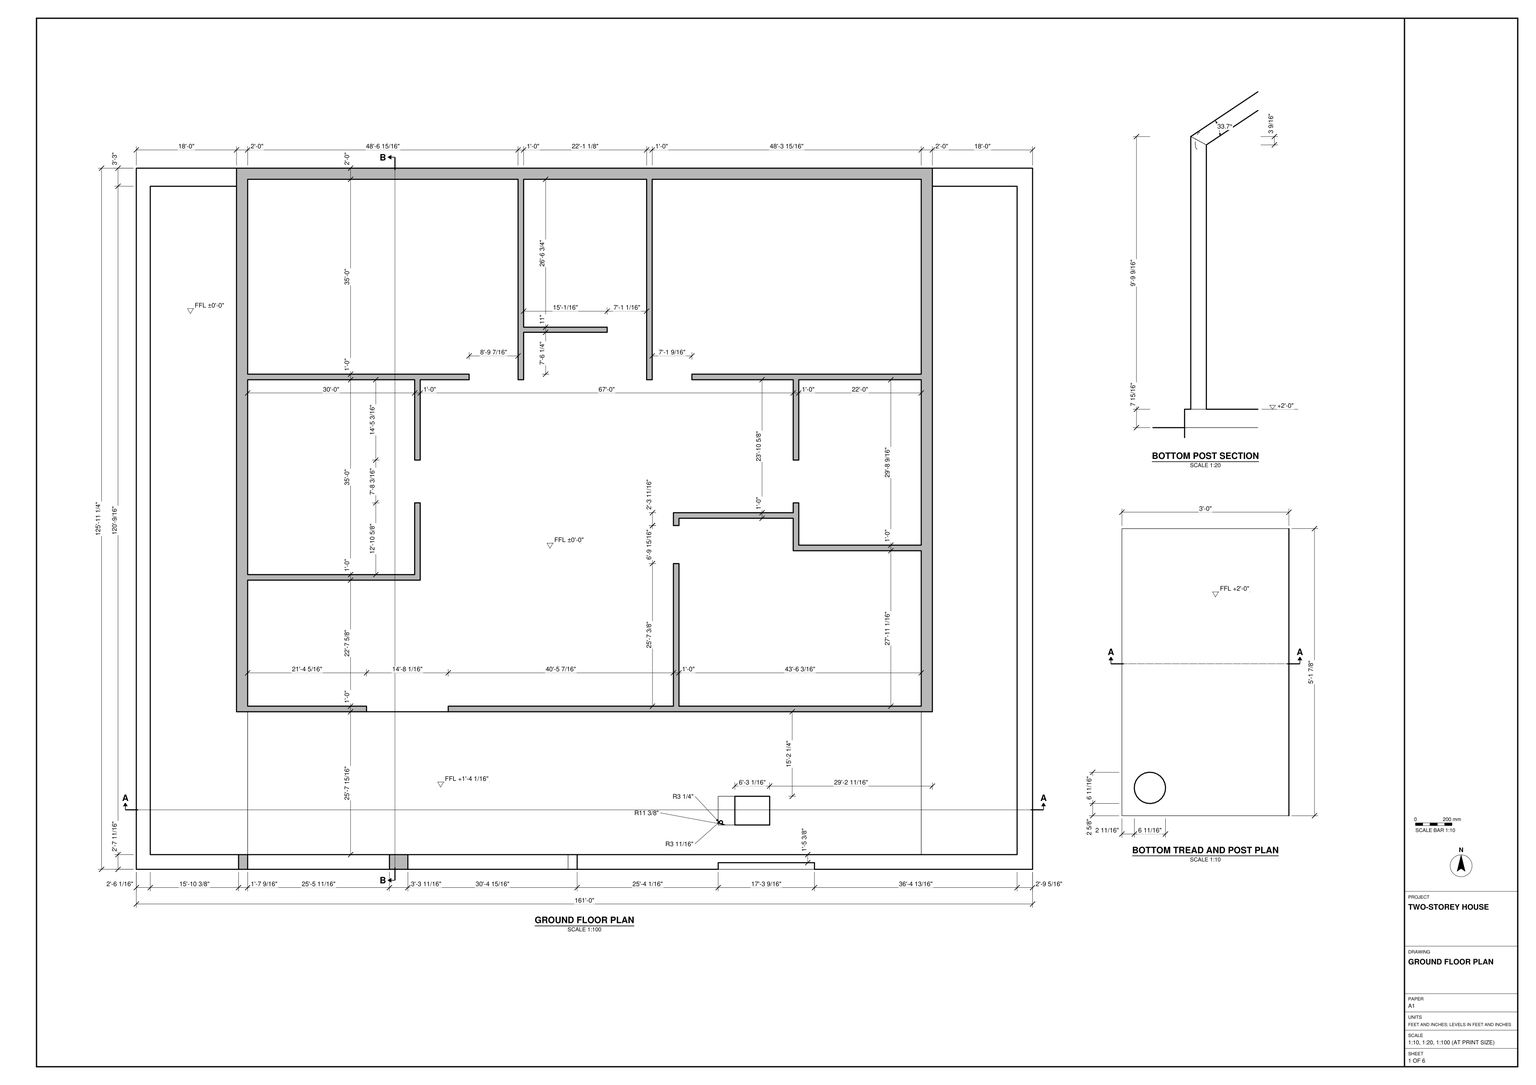
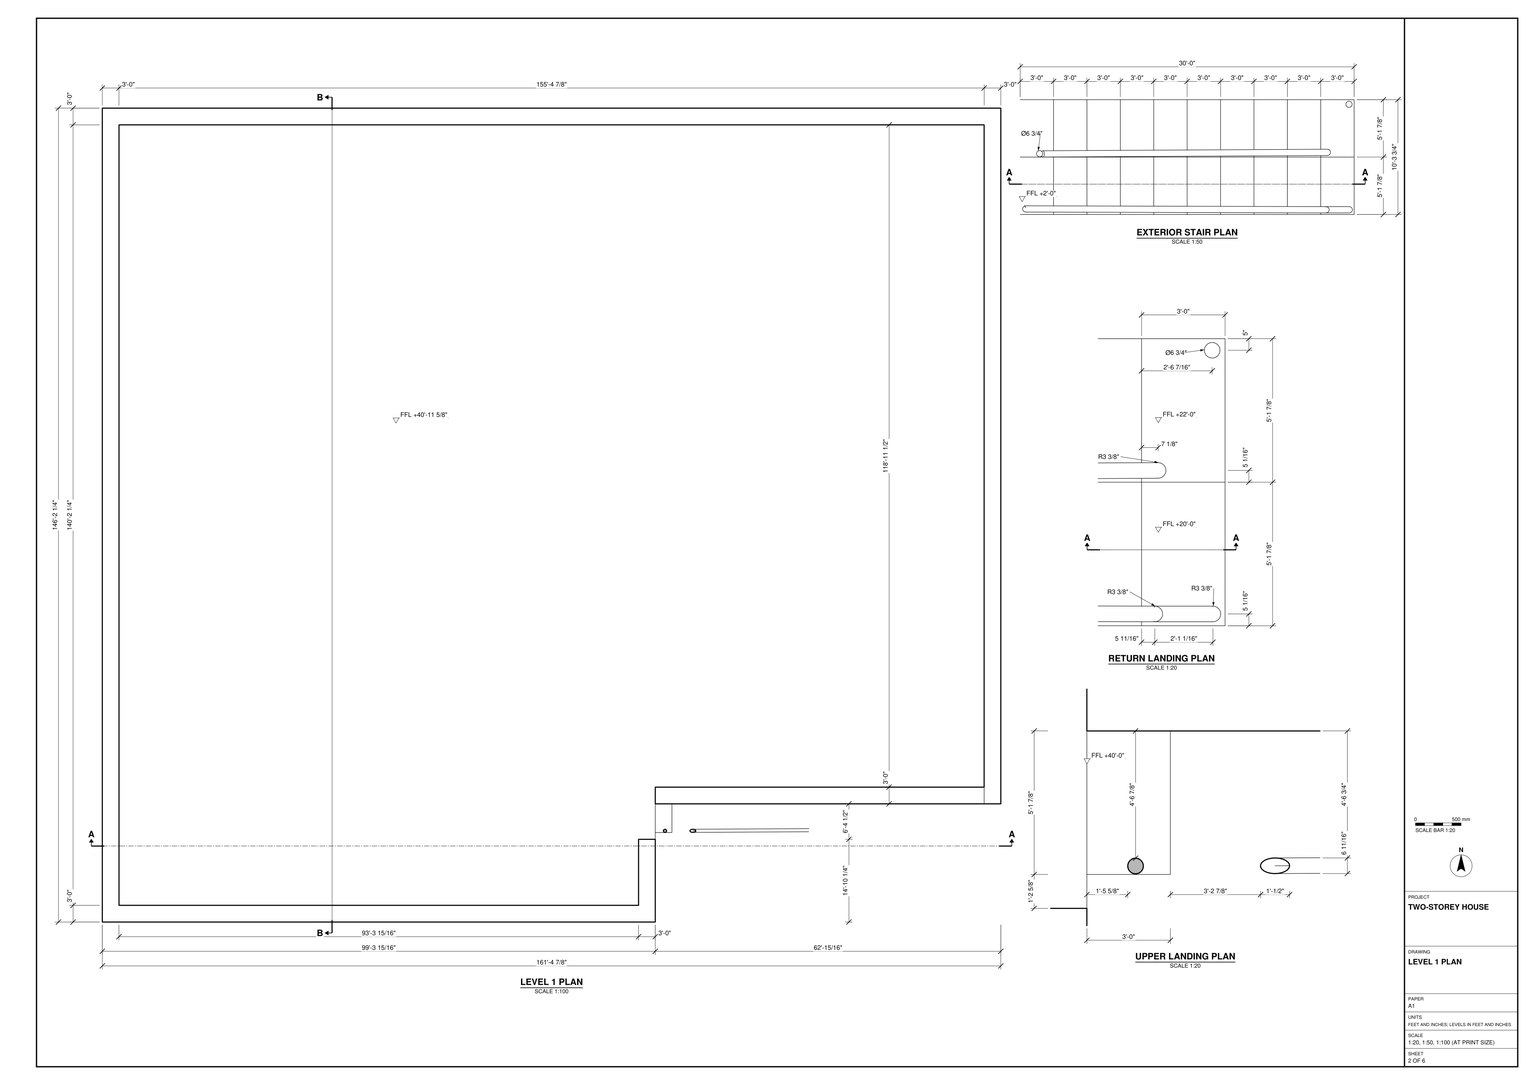
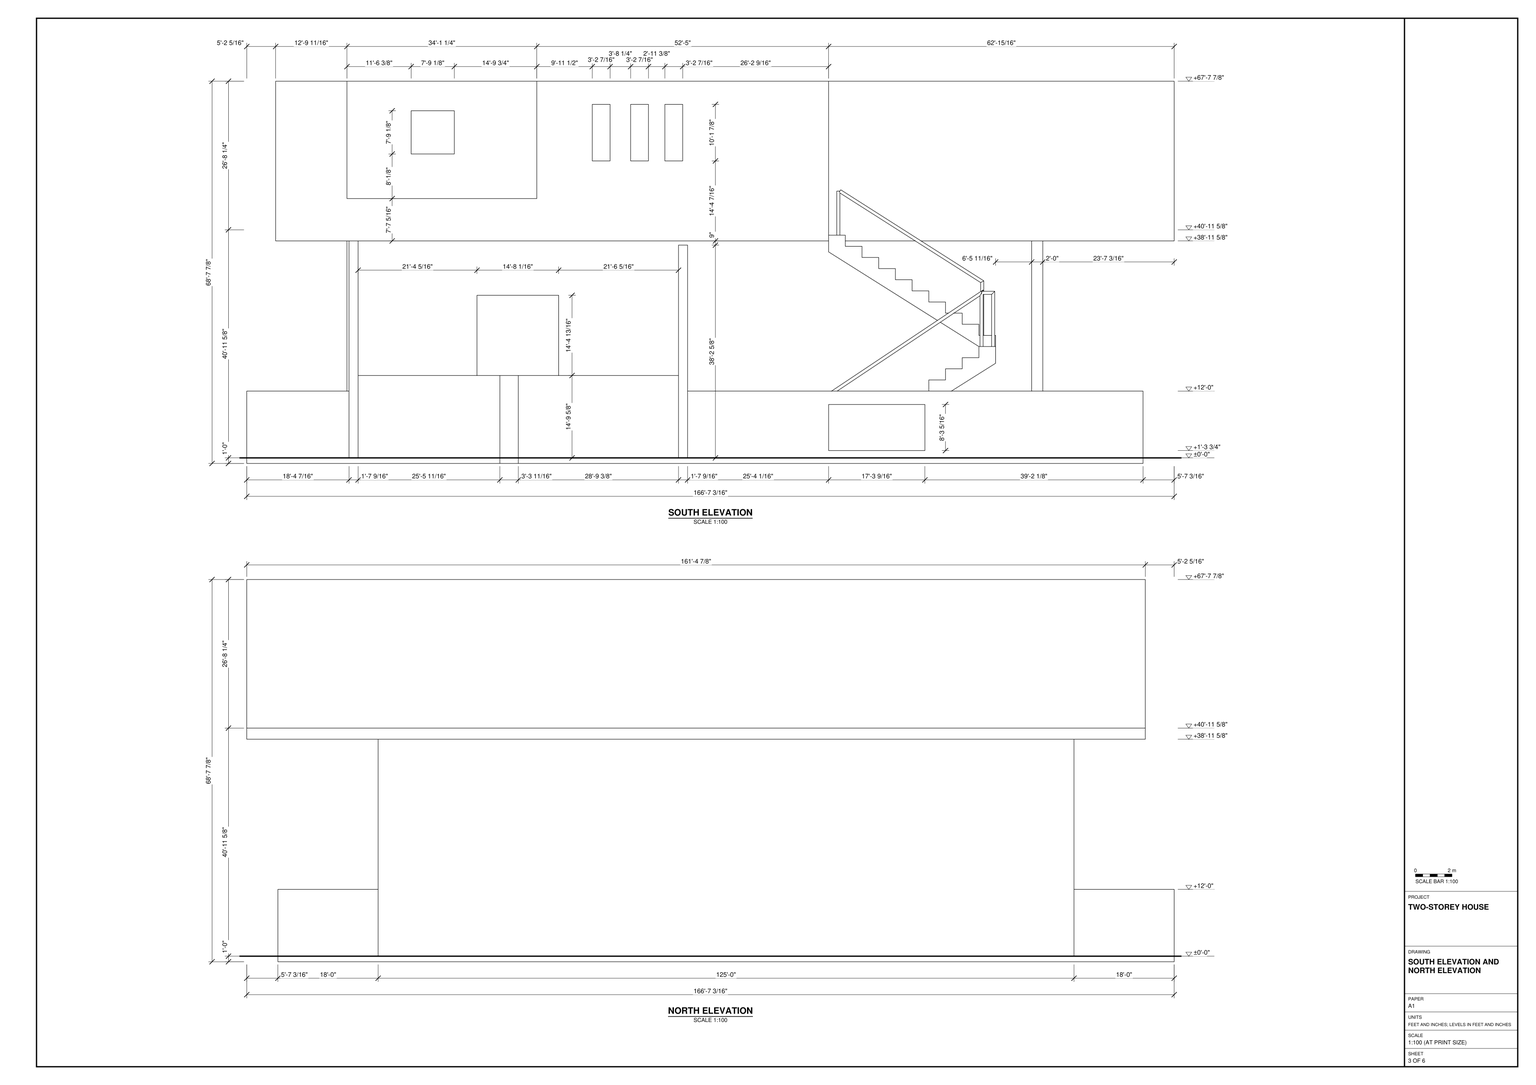
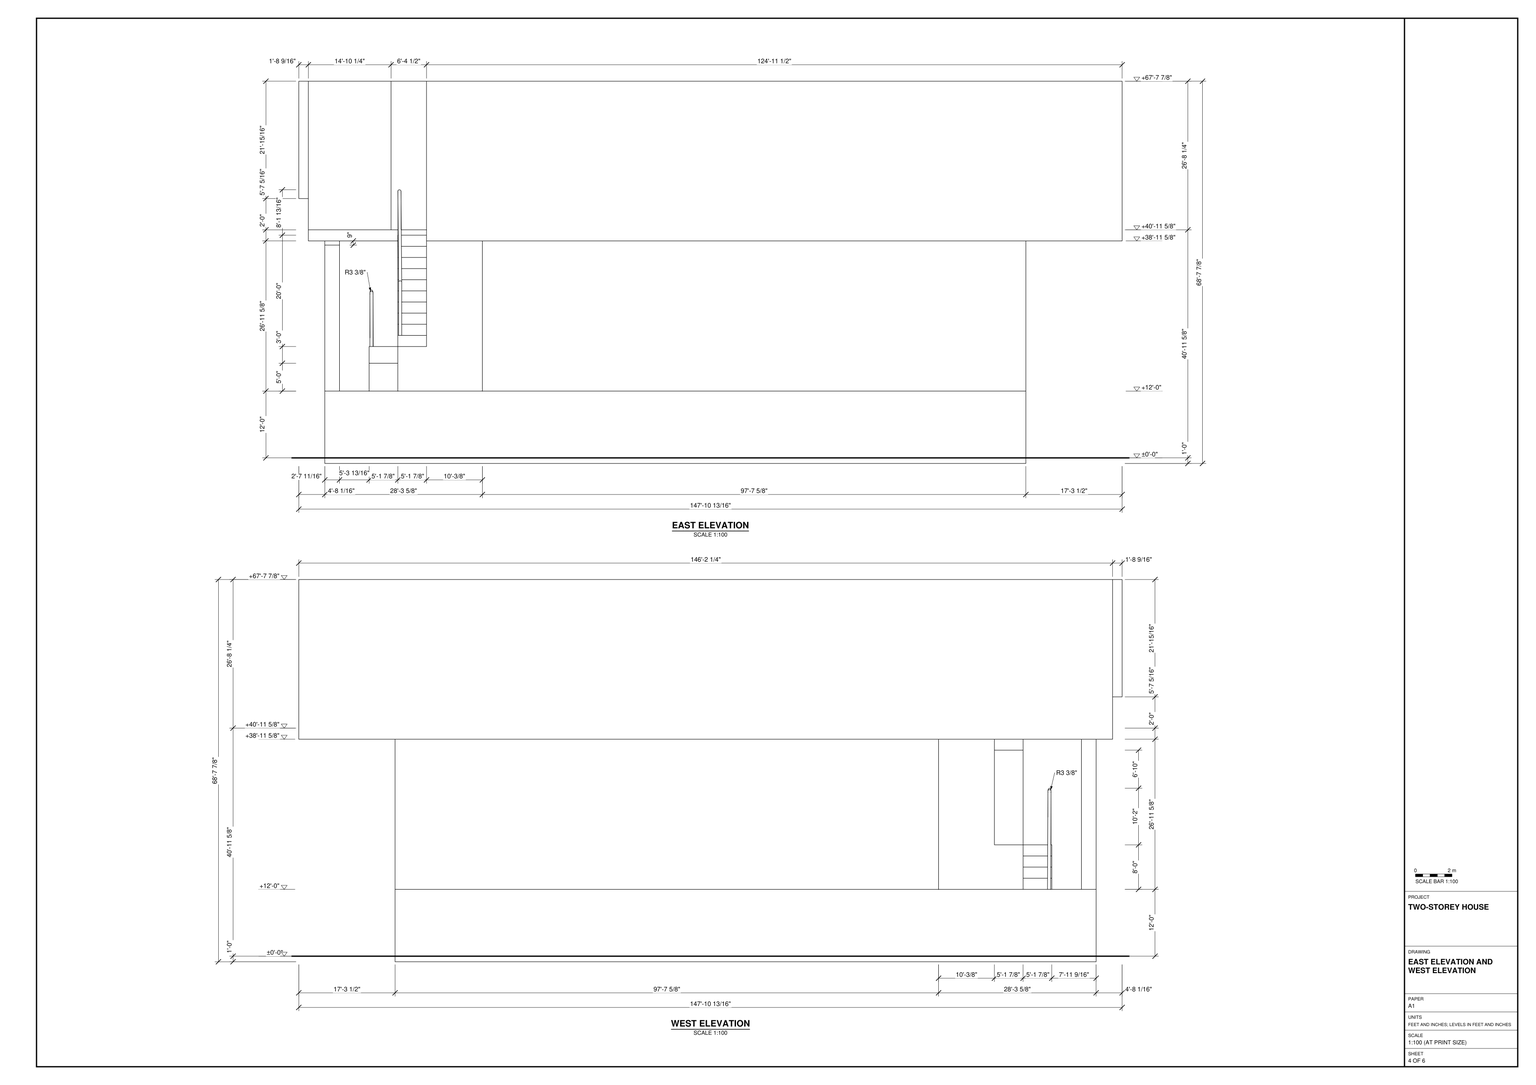
Build the two-storey house shown in task_files/diagram_01.pdf in SketchUp. Work in feet and inches. The overall extents are 166'-7 3/16" along X, 147'-10 13/16" along Y and 68'-7 7/8" along Z. Use ±0'-0" for the ground floor and +40'-11 5/8" for the upper floor.

Lay out the rectangular ground-floor shell, the open strips beside it and the low perimeter wall across the front. Follow the individual wall thicknesses on the plan. Place the internal partitions so that the side rooms connect to the central space through the gaps shown. Form the upper slab with its projecting edges and the rectangular setback at the southeast corner. Use the elevations to place the supports beneath the slab and to set out the square opening and the row of narrow openings on the upper south face. Match the roof profile shown.

Build the exterior stair at the setback, with parallel flights rising in opposite directions. Use the tread, landing and post details to place the handrails. Keep walls, slabs, roof elements and the stair in separate groups or components. Group each furniture or joinery piece shown separately and use components for repeated parts. Any decor or loose items shown may be suitable library components. Save one SketchUp model as output_files/two_storey_house_with_an_exterior_return_stair.skp.

# SketchUp Ruby script. Lengths in inches.
U = 1.inch
M = Sketchup.active_model
def pt(a) = Geom::Point3d.new(a.map { |v| v * U })
def face(e, loops, mat)
  f = e.add_face(loops[0].map { |a| pt(a) })
  loops[1..].each { |l| e.add_face(l.map { |a| pt(a) }).erase! }
  f.material = f.back_material = mat if mat
  f
end
# faces: each face lists its corners as indices into pts; further lists are holes
def faces(e, pts, list, mat = nil) = list.each { |f| face(e, (f[0].is_a?(Array) ? f : [f]).map { |l| l.map { |i| pts[i] } }, mat) }
# xy, xz, yz: faces in a plane at the given z, y or x. An outline is a flat list of corners, or four numbers for a rectangle; further outlines are holes
def ring(l) = l.size == 4 ? [[l[0], l[1]], [l[2], l[1]], [l[2], l[3]], [l[0], l[3]]] : l.each_slice(2).to_a
def flat(e, list, mat, &to3) = list.each { |f| face(e, (f[0].is_a?(Array) ? f : [f]).map { |l| ring(l).map { |u, v| to3.(u, v) } }, mat) }
def xy(e, z, list, mat = nil) = flat(e, list, mat) { |x, y| [x, y, z] }
def xz(e, y, list, mat = nil) = flat(e, list, mat) { |x, z| [x, y, z] }
def yz(e, x, list, mat = nil) = flat(e, list, mat) { |y, z| [x, y, z] }
def lines(e, pts, list) = list.each { |a, b| e.add_line(pt(pts[a]), pt(pts[b])) }
# prism: a flat outline (further loops are holes) pulled along v
def prism(e, loops, v, mat = nil)
  f = face(e, loops, mat); d = Geom::Vector3d.new(v.map { |x| x * U })
  f.pushpull(f.normal.samedirection?(d) ? d.length : -d.length)
end
def box(e, o, s, mat = nil) = prism(e, [[o, [o[0] + s[0], o[1], o[2]], [o[0] + s[0], o[1] + s[1], o[2]], [o[0], o[1] + s[1], o[2]]]], [0, 0, s[2]], mat)
def at(x, y, z, deg = 0) = Geom::Transformation.translation(pt([x, y, z])) * Geom::Transformation.rotation(ORIGIN, Z_AXIS, deg.degrees)
def axes(o, x, y, z) = Geom::Transformation.new([*x, 0, *y, 0, *z, 0, *pt(o).to_a, 1])
def part(name) = M.definitions.add(name)
# library, detail: a bought-in or finely detailed component or shape, given as its bounding box
def library(name, o, s) = part(name).tap { |d| box(d.entities, o, s) }
def detail(e, o, s) = box(e.add_group.entities, o, s)
def put(e, d, t, mat = nil) = e.add_instance(d, t).tap { |i| i.material = mat if mat }
def group(e, t, mat = nil) = e.add_group.tap { |g| g.transformation = t; g.material = mat if mat }.entities
root = M.entities
M.materials.add("[0137_Black]").color = [0, 0, 0]
M.materials.add("[Asphalt New]").color = [67, 60, 62]
M.materials.add("[Blacktop New]").color = [30, 30, 30]
M.materials.add("[Brick Antique 01]").color = [147, 105, 71]
M.materials.add("[Brick Colored Blue]").color = [52, 52, 53]
M.materials.add("[Brick Tumbled]").color = [58, 57, 57]
M.materials.add("[Color A01]").color = [255, 204, 204]
M.materials.add("[Color A08]").color = [48, 0, 0]
M.materials.add("[Color A08]1").color = [40, 0, 0]
M.materials.add("[Color L01]").color = [255, 204, 229]
M.materials.add("[Color M05]").color = [40, 40, 40]
M.materials.add("[Pavers Flagstone Gray]").color = [96, 96, 96]
M.materials.add("[Pavers with Grass Herringbone]").color = [197, 201, 190]
M.materials.add("[Rough Square Concrete Block]").color = [22, 22, 21]
M.materials.add("[Slate Light Tile]").color = [54, 54, 54]
M.materials.add("[Slate]").color = [42, 45, 45]
M.materials.add("[Stone Coursed Rough]").color = [89, 86, 70]
M.materials.add("[Stone Flagstone Ashlar]").color = [175, 116, 102]
M.materials.add("[Terrazzo Tile Accent]").color = [224, 221, 217]
M.materials.add("[Translucent Glass Gray]").color = [128, 128, 128]
M.materials["[Translucent Glass Gray]"].alpha = 0.5
xy(root,0,[[0,56.04,1932,1567.29]])
xy(root,12,[[220.42,56.04,240,87.73],[240,56.04,545.6875,87.73],[545.6875,56.04,585.35,87.73],[585.35,56.04,930.71,87.73],[930.71,56.04,950.29,87.73],
  [950.29,56.04,950.29,87.73,1898.68,87.73,1898.68,1528.29,1716,1528.29,1716,1567.29,1932,1567.29,1932,56.04],[1254.26,151.57,1290.26,213.45],[496.3125,395.6875,672.375,395.6875,672.375,407.6875,1157.8125,407.6875,1157.8125,715.06,1169.8125,715.06,1169.8125,407.6875,1692,407.6875,1692,742.73,1416,742.73,1416,812.6875,1169.8125,812.6875,1169.8125,796.99,1157.8125,796.99,1157.8125,824.6875,1416,824.6875,1416,845.92,1428,845.92,1428,754.73,1692,754.73,1692,1111.29,1428,1111.29,1428,938.12,1416,938.12,1416,1111.29,1197.625,1111.29,1197.625,1123.29,1692,1123.29,1692,1543.29,1112.0625,1543.29,1112.0625,1111.29,1100.0625,1111.29,1100.0625,1543.29,834.9375,1543.29,834.9375,1224.54,1015,1224.54,1015,1213.54,834.9375,1213.54,834.9375,1111.29,822.9375,1111.29,822.9375,1543.29,240,1543.29,240,1123.29,717.47,1123.29,717.47,1111.29,612,1111.29,612,938.12,600,938.12,600,1111.29,240,1111.29,240,691.29,600,691.29,600,845.92,612,845.92,612,679.29,240,679.29,240,407.6875,496.3125,407.6875]])
xy(root,12,[[30.0625,87.73,240,87.73,240,395.6875,216,395.6875,216,1528.29,30.0625,1528.29],[1692,87.73,1898.68,87.73,1898.68,1528.29,1716,1528.29,1716,395.6875,1692,395.6875]],"[Pavers with Grass Herringbone]")
xy(root,27.78,[[1254.33,56.04,1461.89,70.36]])
xy(root,28.0625,[[[240,87.73,1692,395.6875],[1254.26,151.57,1290.26,213.45]]],"[Pavers Flagstone Gray]")
xy(root,36,[[1260.09,154.21,1260.29,154.22,1259.85,154.25],[1260.72,154.25,1260.97,154.27,1261.16,154.33],[1259.42,154.34,1259,154.48,1259.23,154.375],[1261.57,154.47,1261.8,154.56,1261.97,154.66],[1258.61,154.67,1258.25,154.92,1258.44,154.76],
  [1262.33,154.91,1262.53,155.05,1262.66,155.2],[1257.92,155.21,1257.63,155.54,1257.77,155.34],[1262.95,155.53,1263.11,155.71,1263.2,155.89],[1257.39,155.91,1257.2,156.3,1257.28,156.07],[1263.39,156.28,1263.5,156.51,1263.53,156.7],
  [1257.05,156.72,1256.97,157.15,1256.99,156.9],[1263.62,157.13,1263.67,157.37,1263.65,157.57],[1256.94,157.58,1256.97,158.02,1256.93,157.78],[1263.62,158,1263.6,158.25,1263.54,158.43],[1257.06,158.45,1257.2,158.87,1257.09,158.64],
  [1263.4,158.85,1263.32,159.08,1263.21,159.24],[1257.4,159.26,1257.64,159.62,1257.48,159.4375],[1262.96,159.61,1262.82,159.8125,1262.68,159.94],[1257.93,159.95,1258.26,160.24,1258.06,160.1],[1262.34,160.23,1262.16,160.39,1261.98,160.48],
  [1258.625,160.49,1259.02,160.67,1258.79,160.59],[1261.59,160.67,1261.37,160.78,1261.17,160.8125],[1259.4375,160.82,1259.87,160.9,1259.62,160.88],[1260.74,160.9,1260.5,160.94,1260.31,160.93]])
xy(root,36,[[[1254.26,151.57,1290.26,213.45],[1260.48,154.2,1260.29,154.22,1260.09,154.21,1259.85,154.25,1259.6,154.27,1259.42,154.34,1259.23,154.375,1259,154.48,1258.77,154.5625,1258.61,154.67,1258.44,154.76,1258.25,154.92,1258.04,155.0625,1257.92,155.21,1257.77,155.34,1257.63,155.54,1257.47,155.73,1257.39,155.91,1257.28,156.07,1257.2,156.3,1257.09,156.52,1257.05,156.72,1256.99,156.9,1256.97,157.15,1256.93,157.39,1256.94,157.58,1256.93,157.78,1256.97,158.02,1256.99,158.27,1257.06,158.45,1257.09,158.64,1257.2,158.87,1257.29,159.1,1257.4,159.26,1257.48,159.4375,1257.64,159.62,1257.78,159.83,1257.93,159.95,1258.06,160.1,1258.26,160.24,1258.45,160.4,1258.625,160.49,1258.79,160.59,1259.02,160.67,1259.25,160.78,1259.4375,160.82,1259.62,160.88,1259.87,160.9,1260.11,160.94,1260.31,160.93,1260.5,160.94,1260.74,160.9,1260.99,160.88,1261.17,160.8125,1261.37,160.78,1261.59,160.67,1261.82,160.59,1261.98,160.48,1262.16,160.39,1262.34,160.23,1262.55,160.09,1262.68,159.94,1262.82,159.8125,1262.96,159.61,1263.12,159.42,1263.21,159.24,1263.32,159.08,1263.4,158.85,1263.5,158.625,1263.54,158.43,1263.6,158.25,1263.62,158,1263.67,157.76,1263.65,157.57,1263.67,157.37,1263.62,157.13,1263.6,156.88,1263.53,156.7,1263.5,156.51,1263.39,156.28,1263.31,156.05,1263.2,155.89,1263.11,155.71,1262.95,155.53,1262.81,155.32,1262.66,155.2,1262.53,155.05,1262.33,154.91,1262.14,154.75,1261.97,154.66,1261.8,154.56,1261.57,154.47,1261.35,154.37,1261.16,154.33,1260.97,154.27,1260.72,154.25]]],"[Slate Light Tile]")
xy(root,60,[[1290.26,151.57,1326.26,213.45]],"[Slate Light Tile]")
xy(root,84,[[1326.26,151.57,1362.26,213.45]],"[Slate Light Tile]")
xy(root,108,[[1362.26,151.57,1398.26,213.45]],"[Slate Light Tile]")
xy(root,127.09,[[1254.33,56.04,1461.89,70.36]])
xy(root,132,[[1398.26,151.57,1434.26,213.45]],"[Slate Light Tile]")
xy(root,156,[[0,56.04,220.42,56.04,220.42,87.73,30.0625,87.73,30.0625,1528.29,216,1528.29,216,1567.29,0,1567.29],[950.29,56.04,1932,56.04,1932,1567.29,1716,1567.29,1716,1528.29,1898.68,1528.29,1898.68,87.73,950.29,87.73]],"[Brick Antique 01]")
xy(root,156,[[1434.26,151.57,1470.26,213.45]],"[Slate]")
xy(root,180,[[1470.26,151.57,1506.26,213.45]],"[Slate]")
xy(root,189.625,[[545.6875,56.04,585.35,87.73]],"[Blacktop New]")
xy(root,189.625,[[240,56.04,545.6875,87.73],[585.35,56.04,930.71,87.73]],"[Translucent Glass Gray]")
xy(root,204,[[1506.26,151.57,1542.26,213.45]],"[Slate]")
xy(root,228,[[1542.26,151.57,1578.26,213.45]],"[Slate]")
xy(root,252,[[1583.75,153.29,1582.89,153.45,1582.1,153.84,1581.43,154.42,1580.9375,155.15,1580.65,155.98,1580.59,156.86,1580.76,157.72,1581.14,158.52,1581.72,159.18,1582.45,159.68,1583.28,159.96,1584.16,160.02,1585.03,159.86,1585.82,159.47,1586.48,158.89,1586.98,158.16,1587.26,157.33,1587.33,156.45,1587.16,155.59,1586.77,154.79,1586.2,154.13,1585.46,153.64,1584.63,153.35],[1608.82,153.29,1607.95,153.45,1607.16,153.84,1606.49,154.42,1606,155.15,1605.71,155.98,1605.65,156.86,1605.82,157.72,1606.2,158.52,1606.78,159.18,1607.51,159.68,1608.34,159.96,1609.22,160.02,1610.09,159.86,1610.88,159.47,1611.55,158.89,1612.04,158.16,1612.33,157.33,1612.39,156.45,1612.22,155.59,1611.84,154.79,1611.26,154.13,1610.53,153.64,1609.69,153.35],[1578.26,213.45,1614.26,275.32]])
xy(root,252,[[[1578.26,151.57,1614.26,213.45],[1608.82,153.29,1607.95,153.45,1607.16,153.84,1606.49,154.42,1606,155.15,1605.71,155.98,1605.65,156.86,1605.82,157.72,1606.2,158.52,1606.78,159.18,1607.51,159.68,1608.34,159.96,1609.22,160.02,1610.09,159.86,1610.88,159.47,1611.55,158.89,1612.04,158.16,1612.33,157.33,1612.39,156.45,1612.22,155.59,1611.84,154.79,1611.26,154.13,1610.53,153.64,1609.69,153.35],[1583.75,153.29,1582.89,153.45,1582.1,153.84,1581.43,154.42,1580.9375,155.15,1580.65,155.98,1580.59,156.86,1580.76,157.72,1581.14,158.52,1581.72,159.18,1582.45,159.68,1583.28,159.96,1584.16,160.02,1585.03,159.86,1585.82,159.47,1586.48,158.89,1586.98,158.16,1587.26,157.33,1587.33,156.45,1587.16,155.59,1586.77,154.79,1586.2,154.13,1585.46,153.64,1584.63,153.35]]],"[Slate]")
xy(root,276,[[1585.19,215.16,1584.33,215.33,1583.54,215.72,1582.87,216.29,1582.38,217.02,1582.09,217.86,1582.03,218.73,1582.2,219.6,1582.58,220.39,1583.16,221.06,1583.89,221.55,1584.72,221.84,1585.6,221.9,1586.47,221.73,1587.26,221.35,1587.92,220.77,1588.42,220.04,1588.7,219.21,1588.77,218.33,1588.6,217.46,1588.21,216.67,1587.64,216,1586.91,215.51,1586.07,215.22]])
xy(root,276,[[1608.5,266.96,1609.38,267.02,1610.22,267.31,1610.95,267.8,1611.52,268.46,1611.91,269.26,1612.08,270.12,1612.02,271,1611.73,271.83,1611.23,272.5625,1610.57,273.14,1609.78,273.53,1608.91,273.69,1608.03,273.63,1607.2,273.34,1606.47,272.85,1605.89,272.1875,1605.51,271.39,1605.34,270.53,1605.4,269.65,1605.6875,268.82,1606.18,268.09,1606.85,267.51,1607.64,267.125]],"[Slate Light Tile]")
xy(root,276,[[[1578.26,213.45,1614.26,275.32],[1608.5,266.96,1607.64,267.125,1606.85,267.51,1606.18,268.09,1605.6875,268.82,1605.4,269.65,1605.34,270.53,1605.51,271.39,1605.89,272.1875,1606.47,272.85,1607.2,273.34,1608.03,273.63,1608.91,273.69,1609.78,273.53,1610.57,273.14,1611.23,272.5625,1611.73,271.83,1612.02,271,1612.08,270.12,1611.91,269.26,1611.52,268.46,1610.95,267.8,1610.22,267.31,1609.38,267.02],[1585.19,215.16,1584.33,215.33,1583.54,215.72,1582.87,216.29,1582.38,217.02,1582.09,217.86,1582.03,218.73,1582.2,219.6,1582.58,220.39,1583.16,221.06,1583.89,221.55,1584.72,221.84,1585.6,221.9,1586.47,221.73,1587.26,221.35,1587.92,220.77,1588.42,220.04,1588.7,219.21,1588.77,218.33,1588.6,217.46,1588.21,216.67,1587.64,216,1586.91,215.51,1586.07,215.22]]],"[Slate]")
xy(root,300,[[1542.26,213.45,1578.26,275.32]],"[Slate]")
xy(root,324,[[1506.26,213.45,1542.26,275.32]],"[Slate]")
xy(root,348,[[1470.26,213.45,1506.26,275.32]],"[Slate]")
xy(root,362.4375,[[496.3125,395.6875,672.375,407.6875]])
xy(root,372,[[1434.26,213.45,1470.26,275.32]],"[Slate]")
xy(root,396,[[1398.26,213.45,1434.26,275.32]],"[Slate]")
xy(root,420,[[1362.26,213.45,1398.26,275.32]],"[Slate]")
xy(root,444,[[1326.26,213.45,1362.26,275.32]],"[Slate]")
xy(root,468,[[1290.26,213.45,1326.26,275.32]],"[Slate]")
xy(root,470.625,[[930.71,56.04,950.29,87.73]])
xy(root,479.625,[[62.3125,20.5625,216,1774.8125],[216,20.5625,1254.26,395.6875],[220.42,56.04,240,87.73],[1254.26,275.3125,1716,395.6875],[1716,275.3125,1999.1875,311.3125],
  [1716,311.3125,1999.1875,395.6875],[216,395.6875,496.3125,395.6875,496.3125,407.6875,240,407.6875,240,679.29,612,679.29,612,845.92,600,845.92,600,691.29,240,691.29,240,1111.29,600,1111.29,600,938.12,612,938.12,612,1111.29,717.47,1111.29,717.47,1123.29,240,1123.29,240,1543.29,822.9375,1543.29,822.9375,1111.29,834.9375,1111.29,834.9375,1213.54,1015,1213.54,1015,1224.54,834.9375,1224.54,834.9375,1543.29,1100.0625,1543.29,1100.0625,1111.29,1112.0625,1111.29,1112.0625,1543.29,1692,1543.29,1692,1123.29,1197.625,1123.29,1197.625,1111.29,1416,1111.29,1416,938.12,1428,938.12,1428,1111.29,1692,1111.29,1692,754.73,1428,754.73,1428,845.92,1416,845.92,1416,824.6875,1157.8125,824.6875,1157.8125,796.99,1169.8125,796.99,1169.8125,812.6875,1416,812.6875,1416,742.73,1692,742.73,1692,407.6875,1169.8125,407.6875,1169.8125,715.06,1157.8125,715.06,1157.8125,407.6875,672.375,407.6875,672.375,395.6875,1716,395.6875,1716,1567.29,216,1567.29],[496.3125,395.6875,672.375,407.6875],[1716,395.6875,1999.1875,1774.8125],[240,407.6875,240,679.29,612,679.29,612,845.92,600,845.92,600,691.29,240,691.29,240,1111.29,600,1111.29,600,938.12,612,938.12,612,1111.29,717.47,1111.29,717.47,1123.29,240,1123.29,240,1543.29,822.9375,1543.29,822.9375,1111.29,834.9375,1111.29,834.9375,1213.54,1015,1213.54,1015,1224.54,834.9375,1224.54,834.9375,1543.29,1100.0625,1543.29,1100.0625,1111.29,1112.0625,1111.29,1112.0625,1543.29,1692,1543.29,1692,1123.29,1197.625,1123.29,1197.625,1111.29,1416,1111.29,1416,938.12,1428,938.12,1428,1111.29,1692,1111.29,1692,754.73,1428,754.73,1428,845.92,1416,845.92,1416,824.6875,1157.8125,824.6875,1157.8125,796.99,1169.8125,796.99,1169.8125,812.6875,1416,812.6875,1416,742.73,1692,742.73,1692,407.6875,1169.8125,407.6875,1169.8125,715.06,1157.8125,715.06,1157.8125,407.6875],
  [216,1567.29,1716,1774.8125]])
xy(root,492,[[1275.05,213.72,1274.1875,213.89,1273.4,214.28,1272.73,214.86,1272.24,215.59,1271.95,216.42,1271.89,217.3,1272.06,218.16,1272.44,218.95,1273.02,219.62,1273.75,220.11,1274.58,220.4,1275.46,220.46,1276.33,220.29,1277.12,219.91,1277.78,219.33,1278.28,218.6,1278.5625,217.77,1278.625,216.89,1278.46,216.02,1278.07,215.23,1277.5,214.57,1276.77,214.07,1275.93,213.79]])
xy(root,492,[[[1254.26,213.45,1290.26,275.32],[1275.05,213.72,1274.1875,213.89,1273.4,214.28,1272.73,214.86,1272.24,215.59,1271.95,216.42,1271.89,217.3,1272.06,218.16,1272.44,218.95,1273.02,219.62,1273.75,220.11,1274.58,220.4,1275.46,220.46,1276.33,220.29,1277.12,219.91,1277.78,219.33,1278.28,218.6,1278.5625,217.77,1278.625,216.89,1278.46,216.02,1278.07,215.23,1277.5,214.57,1276.77,214.07,1275.93,213.79]]],"[Slate]")
xy(root,503.625,[[98.3125,56.5625,1218.26,56.5625,1218.26,198.84,1254.26,198.84,1254.26,311.3125,1963.1875,311.3125,1963.1875,1738.8125,98.3125,1738.8125]])
xy(root,570.9375,[[216,0,625.26,20.5625]])
xy(root,587,[[1275.05,213.72,1275.93,213.79,1276.77,214.07,1277.5,214.57,1278.07,215.23,1278.46,216.02,1278.625,216.89,1278.5625,217.77,1278.28,218.6,1277.78,219.33,1277.12,219.91,1276.33,220.29,1275.46,220.46,1274.58,220.4,1273.75,220.11,1273.02,219.62,1272.44,218.95,1272.06,218.16,1271.89,217.3,1271.95,216.42,1272.24,215.59,1272.73,214.86,1273.4,214.28,1274.1875,213.89]],"[Slate Light Tile]")
xy(root,652.09,[[744.79,20.5625,783.23,56.5625],[827.48,20.5625,865.92,56.5625],[901.29,20.5625,939.73,56.5625]])
xy(root,773.97,[[744.79,20.5625,783.23,56.5625],[827.48,20.5625,865.92,56.5625],[901.29,20.5625,939.73,56.5625]])
xy(root,823.875,[[216,0,625.26,0,625.26,20.5625,1254.26,20.5625,1254.26,198.84,1218.26,198.84,1218.26,56.5625,98.3125,56.5625,98.3125,1738.8125,1963.1875,1738.8125,1963.1875,311.3125,1254.26,311.3125,1254.26,275.3125,1999.1875,275.3125,1999.1875,1774.8125,62.3125,1774.8125,62.3125,20.5625,216,20.5625]],"[Brick Colored Blue]")
xz(root,0,[[[216,570.9375,625.26,823.875],[354.36,667.0625,447.48,760.1875]]],"[Asphalt New]")
xz(root,20.5625,[[[62.3125,479.625,1254.26,479.625,1254.26,823.875,625.26,823.875,625.26,570.9375,216,570.9375,216,823.875,62.3125,823.875],[901.29,652.09,939.73,773.97],[827.48,652.09,865.92,773.97],[744.79,652.09,783.23,773.97]]],"[Color M05]")
xz(root,56.04,[[545.6875,0,585.35,12]])
xz(root,56.04,[[545.6875,12,585.35,189.625]],"[Blacktop New]")
xz(root,56.04,[[0,0,545.6875,12],[585.35,0,1932,12],[0,12,220.42,156],[[950.29,12,1932,156],[1254.33,27.78,1461.89,127.09]]],"[Brick Antique 01]")
xz(root,56.04,[[220.42,12,240,479.625],[930.71,12,950.29,470.625]],"[Color L01]")
xz(root,56.04,[[240,12,545.6875,189.625],[585.35,12,930.71,189.625]],"[Translucent Glass Gray]")
xz(root,56.5625,[[[98.3125,503.625,1218.26,823.875],[901.29,652.09,939.73,773.97],[827.48,652.09,865.92,773.97],[744.79,652.09,783.23,773.97]]],"[Terrazzo Tile Accent]")
xz(root,70.36,[[1254.33,27.78,1461.89,127.09]],"[Stone Flagstone Ashlar]")
xz(root,87.73,[[30.0625,12,220.42,156],[220.42,12,240,479.625],[240,12,545.6875,28.0625],[545.6875,12,585.35,28.0625],[585.35,12,930.71,28.0625],
  [930.71,12,950.29,28.0625],[950.29,12,1692,28.0625],[545.6875,28.0625,585.35,189.625],[930.71,28.0625,950.29,470.625]])
xz(root,87.73,[[1692,12,1898.68,156],[950.29,28.0625,1692,156]],"[Brick Antique 01]")
xz(root,87.73,[[240,28.0625,545.6875,189.625],[585.35,28.0625,930.71,189.625]],"[Translucent Glass Gray]")
xz(root,151.57,[[1254.26,12,1290.26,28.0625]])
xz(root,151.57,[[1290.26,12,1614.26,216,1614.26,252,1578.26,252,1578.26,228,1542.26,228,1542.26,204,1506.26,204,1506.26,180,1470.26,180,1470.26,156,1434.26,156,1434.26,132,1398.26,132,1398.26,108,1362.26,108,1362.26,84,1326.26,84,1326.26,60,1290.26,60,1290.26,36,1254.26,36,1254.26,28.0625,1290.26,28.0625]],"[Slate]")
xz(root,198.84,[[1218.26,503.625,1254.26,823.875]])
xz(root,213.45,[[1254.26,12,1290.26,28.0625],[1290.26,12,1290.26,28.0625,1254.26,28.0625,1254.26,36,1290.26,36,1290.26,60,1326.26,60,1326.26,84,1362.26,84,1362.26,108,1398.26,108,1398.26,132,1434.26,132,1434.26,156,1470.26,156,1470.26,180,1506.26,180,1506.26,204,1542.26,204,1542.26,228,1578.26,228,1578.26,252,1614.26,252,1614.26,216]])
xz(root,213.45,[[1578.26,252,1614.26,252,1614.26,276,1578.26,276,1578.26,300,1542.26,300,1542.26,324,1506.26,324,1506.26,348,1470.26,348,1470.26,372,1434.26,372,1434.26,396,1398.26,396,1398.26,420,1362.26,420,1362.26,444,1326.26,444,1326.26,468,1290.26,468,1290.26,492,1254.26,492,1254.26,456]],"[Slate]")
xz(root,275.3125,[[1254.26,479.625,1999.1875,823.875]],"[Color M05]")
xz(root,275.32,[[1578.26,252,1254.26,456,1254.26,492,1290.26,492,1290.26,468,1326.26,468,1326.26,444,1362.26,444,1362.26,420,1398.26,420,1398.26,396,1434.26,396,1434.26,372,1470.26,372,1470.26,348,1506.26,348,1506.26,324,1542.26,324,1542.26,300,1578.26,300,1578.26,276,1614.26,276,1614.26,252]])
xz(root,311.3125,[[1254.26,503.625,1963.1875,823.875]])
xz(root,395.6875,[[240,12,496.3125,28.0625],[496.3125,12,672.375,28.0625],[672.375,12,1692,28.0625]])
xz(root,395.6875,[[496.3125,28.0625,672.375,362.4375]],"[Color A08]1")
xz(root,395.6875,[[216,12,240,479.625],[1692,12,1716,479.625]],"[Rough Square Concrete Block]")
xz(root,395.6875,[[240,28.0625,496.3125,28.0625,496.3125,362.4375,672.375,362.4375,672.375,28.0625,1692,28.0625,1692,479.625,240,479.625]],"[Stone Coursed Rough]")
xz(root,407.6875,[[240,12,496.3125,479.625],[672.375,12,1157.8125,479.625],[1169.8125,12,1692,479.625],[496.3125,362.4375,672.375,479.625]])
xz(root,679.29,[[240,12,612,479.625]],"[Color A08]")
xz(root,691.29,[[240,12,600,479.625]])
xz(root,715.06,[[1157.8125,12,1169.8125,479.625]])
xz(root,742.73,[[1416,12,1692,479.625]])
xz(root,754.73,[[1428,12,1692,479.625]])
xz(root,796.99,[[1157.8125,12,1169.8125,479.625]])
xz(root,812.6875,[[1169.8125,12,1416,479.625]])
xz(root,824.6875,[[1157.8125,12,1416,479.625]])
xz(root,845.92,[[600,12,612,479.625],[1416,12,1428,479.625]])
xz(root,938.12,[[600,12,612,479.625],[1416,12,1428,479.625]])
xz(root,1111.29,[[240,12,600,479.625],[822.9375,12,834.9375,479.625],[1100.0625,12,1112.0625,479.625],[1197.625,12,1416,479.625],[1428,12,1692,479.625]])
xz(root,1111.29,[[612,12,717.47,479.625]],"[Color A08]")
xz(root,1123.29,[[240,12,717.47,479.625],[1197.625,12,1692,479.625]])
xz(root,1213.54,[[834.9375,12,1015,479.625]])
xz(root,1224.54,[[834.9375,12,1015,479.625]])
xz(root,1528.29,[[30.0625,12,216,156],[1716,12,1898.68,156]],"[Brick Antique 01]")
xz(root,1543.29,[[240,12,822.9375,479.625],[834.9375,12,1100.0625,479.625],[1112.0625,12,1692,479.625]])
xz(root,1567.29,[[0,12,216,156],[1716,12,1932,156]],"[Brick Antique 01]")
xz(root,1567.29,[[0,0,0,12,216,12,216,479.625,1716,479.625,1716,12,1932,12,1932,0]],"[Color A01]")
xz(root,1738.8125,[[98.3125,503.625,1963.1875,823.875]])
xz(root,1774.8125,[[62.3125,479.625,1999.1875,503.625]])
xz(root,1774.8125,[[62.3125,503.625,1999.1875,823.875]],"[Brick Tumbled]")
yz(root,0,[[56.04,0,1567.29,156]],"[Brick Antique 01]")
yz(root,30.0625,[[87.73,12,1528.29,156]],"[Brick Antique 01]")
yz(root,62.3125,[[20.5625,479.625,1774.8125,823.875]],"[Brick Colored Blue]")
yz(root,98.3125,[[56.5625,503.625,1738.8125,823.875]])
yz(root,216,[[1528.29,12,1567.29,156]])
yz(root,216,[[0,570.9375,20.5625,823.875]],"[Brick Colored Blue]")
yz(root,216,[[395.6875,12,395.6875,479.625,1567.29,479.625,1567.29,156,1528.29,156,1528.29,12]],"[Color A01]")
yz(root,220.42,[[56.04,12,87.73,156]])
yz(root,220.42,[[56.04,156,87.73,479.625]],"[Color L01]")
yz(root,240,[[56.04,12,87.73,189.625],[407.6875,12,679.29,479.625],[691.29,12,1111.29,479.625],[1123.29,12,1543.29,479.625]])
yz(root,240,[[56.04,189.625,87.73,479.625]],"[Color L01]")
yz(root,240,[[87.73,12,395.6875,28.0625]],"[Pavers Flagstone Gray]")
yz(root,496.3125,[[395.6875,12,407.6875,362.4375]])
yz(root,545.6875,[[56.04,12,87.73,189.625]])
yz(root,585.35,[[56.04,12,87.73,189.625]])
yz(root,600,[[691.29,12,845.92,479.625],[938.12,12,1111.29,479.625]])
yz(root,612,[[679.29,12,845.92,479.625],[938.12,12,1111.29,479.625]])
yz(root,625.26,[[0,570.9375,20.5625,823.875]])
yz(root,672.375,[[395.6875,12,407.6875,362.4375]])
yz(root,717.47,[[1111.29,12,1123.29,479.625]])
yz(root,744.79,[[20.5625,652.09,56.5625,773.97]])
yz(root,783.23,[[20.5625,652.09,56.5625,773.97]])
yz(root,822.9375,[[1111.29,12,1543.29,479.625]])
yz(root,827.48,[[20.5625,652.09,56.5625,773.97]])
yz(root,834.9375,[[1111.29,12,1213.54,479.625],[1224.54,12,1543.29,479.625]])
yz(root,865.92,[[20.5625,652.09,56.5625,773.97]])
yz(root,901.29,[[20.5625,652.09,56.5625,773.97]])
yz(root,930.71,[[56.04,189.625,87.73,470.625]],"[Color L01]")
yz(root,939.73,[[20.5625,652.09,56.5625,773.97]])
yz(root,950.29,[[56.04,12,87.73,156]])
yz(root,950.29,[[56.04,156,87.73,470.625]],"[Color L01]")
yz(root,1015,[[1213.54,12,1224.54,479.625]])
yz(root,1100.0625,[[1111.29,12,1543.29,479.625]])
yz(root,1112.0625,[[1111.29,12,1543.29,479.625]])
yz(root,1157.8125,[[407.6875,12,715.06,479.625],[796.99,12,824.6875,479.625]])
yz(root,1169.8125,[[407.6875,12,715.06,479.625],[796.99,12,812.6875,479.625]])
yz(root,1197.625,[[1111.29,12,1123.29,479.625]])
yz(root,1218.26,[[56.5625,503.625,198.84,823.875]])
yz(root,1254.26,[[151.57,12,213.45,28.0625],[213.45,456,275.32,479.625],[213.45,479.625,275.3125,492],[275.3125,479.625,275.32,492],[275.3125,503.625,311.3125,823.875]])
yz(root,1254.26,[[20.5625,479.625,213.45,479.625,213.45,492,275.3125,492,275.3125,503.625,20.5625,503.625],[20.5625,503.625,198.84,823.875]],"[Rough Square Concrete Block]")
yz(root,1254.26,[[151.57,28.0625,213.45,36]],"[Slate Light Tile]")
yz(root,1254.33,[[56.04,27.78,70.36,127.09]])
yz(root,1290.26,[[151.57,12,213.45,28.0625]])
yz(root,1290.26,[[151.57,36,213.45,60]],"[Slate Light Tile]")
yz(root,1290.26,[[213.45,468,275.32,492]],"[Slate]")
yz(root,1326.26,[[151.57,60,213.45,84]],"[Slate Light Tile]")
yz(root,1326.26,[[213.45,444,275.32,468]],"[Slate]")
yz(root,1362.26,[[151.57,84,213.45,108]],"[Slate Light Tile]")
yz(root,1362.26,[[213.45,420,275.32,444]],"[Slate]")
yz(root,1398.26,[[151.57,108,213.45,132]],"[Slate Light Tile]")
yz(root,1398.26,[[213.45,396,275.32,420]],"[Slate]")
yz(root,1416,[[742.73,12,812.6875,479.625],[824.6875,12,845.92,479.625],[938.12,12,1111.29,479.625]])
yz(root,1428,[[754.73,12,845.92,479.625],[938.12,12,1111.29,479.625]])
yz(root,1434.26,[[151.57,132,213.45,156]],"[Slate Light Tile]")
yz(root,1434.26,[[213.45,372,275.32,396]],"[Slate]")
yz(root,1461.89,[[56.04,27.78,70.36,127.09]])
yz(root,1470.26,[[151.57,156,213.45,180]],"[Slate Light Tile]")
yz(root,1470.26,[[213.45,348,275.32,372]],"[Slate]")
yz(root,1506.26,[[151.57,180,213.45,204]],"[Slate Light Tile]")
yz(root,1506.26,[[213.45,324,275.32,348]],"[Slate]")
yz(root,1542.26,[[151.57,204,213.45,228]],"[Slate Light Tile]")
yz(root,1542.26,[[213.45,300,275.32,324]],"[Slate]")
yz(root,1578.26,[[151.57,228,213.45,252]],"[Slate Light Tile]")
yz(root,1578.26,[[213.45,276,275.32,300]],"[Slate]")
yz(root,1583.96,[[156.86,364.38,156.66,364.4,155.98,364.44,155.15,364.73,154.42,365.22,153.84,365.89,153.45,366.68,153.29,367.55,153.35,368.43,153.64,369.26,154.13,369.99,154.79,370.57,155.59,370.95,156.45,371.12,157.33,371.06,158.16,370.77,158.89,370.28,159.47,369.61,159.86,368.82,160.02,367.95,159.96,367.07,159.68,366.24,159.18,365.51,158.52,364.93,157.72,364.55]])
yz(root,1614.26,[[151.57,216,213.45,252],[213.45,252,275.32,276]],"[Slate]")
yz(root,1692,[[407.6875,12,742.73,479.625],[754.73,12,1111.29,479.625],[1123.29,12,1543.29,479.625]])
yz(root,1692,[[87.73,12,395.6875,28.0625]],"[Pavers Flagstone Gray]")
yz(root,1716,[[1528.29,12,1567.29,156]])
yz(root,1716,[[395.6875,12,1528.29,12,1528.29,156,1567.29,156,1567.29,479.625,395.6875,479.625]],"[Color A01]")
yz(root,1898.68,[[87.73,12,1528.29,156]],"[Brick Antique 01]")
yz(root,1932,[[56.04,0,1567.29,12],[56.04,12,1567.29,156]],"[Brick Antique 01]")
yz(root,1963.1875,[[311.3125,503.625,1738.8125,823.875]])
yz(root,1999.1875,[[275.3125,479.625,1774.8125,823.875]],"[Brick Colored Blue]")
p = [[1614.26,151.57,216],[1290.26,151.57,12],[1290.26,213.45,12],[1614.26,213.45,216],[1260.48,154.2,151.65],[1259.6,154.27,152.12],
  [1259.6,154.27,36],[1259.85,154.25,36],[1260.29,154.22,36],[1260.48,154.2,36],[1261.35,154.37,151.18],[1260.72,154.25,36],
  [1261.16,154.33,36],[1261.35,154.37,36],[1258.77,154.5625,152.5625],[1258.77,154.5625,36],[1259,154.48,36],[1259.42,154.34,36],
  [1262.14,154.75,150.76],[1261.57,154.47,36],[1261.97,154.66,36],[1262.14,154.75,36],[1258.04,155.0625,152.95],[1258.04,155.0625,36],
  [1258.25,154.92,36],[1258.61,154.67,36],[1262.81,155.32,150.4],[1262.33,154.91,36],[1262.66,155.2,36],[1262.81,155.32,36],
  [1257.47,155.73,153.26],[1257.47,155.73,36],[1257.63,155.54,36],[1257.92,155.21,36],[1263.31,156.05,150.14],[1262.95,155.53,36],
  [1263.2,155.89,36],[1263.31,156.05,36],[1257.09,156.52,153.46],[1257.09,156.52,36],[1257.2,156.3,36],[1257.39,155.91,36],
  [1263.6,156.88,149.98],[1263.39,156.28,36],[1263.53,156.7,36],[1263.6,156.88,36],[1256.93,157.39,153.55],[1256.93,157.39,36],
  [1256.97,157.15,36],[1257.05,156.72,36],[1263.67,157.76,149.95],[1263.62,157.13,36],[1263.65,157.57,36],[1263.67,157.76,36],
  [1256.99,158.27,153.52],[1256.99,158.27,36],[1256.97,158.02,36],[1256.94,157.58,36],[1263.5,158.625,150.04],[1263.62,158,36],
  [1263.54,158.43,36],[1263.5,158.625,36],[1257.29,159.1,153.36],[1257.29,159.1,36],[1257.2,158.87,36],[1257.06,158.45,36],
  [1263.12,159.42,150.24],[1263.4,158.85,36],[1263.21,159.24,36],[1263.12,159.42,36],[1257.78,159.83,153.1],[1257.78,159.83,36],
  [1257.64,159.62,36],[1257.4,159.26,36],[1262.55,160.09,150.55],[1262.96,159.61,36],[1262.68,159.94,36],[1262.55,160.09,36],
  [1258.45,160.4,152.74],[1258.45,160.4,36],[1258.26,160.24,36],[1257.93,159.95,36],[1261.82,160.59,150.9375],[1262.34,160.23,36],
  [1261.98,160.48,36],[1261.82,160.59,36],[1259.25,160.78,152.32],[1259.25,160.78,36],[1259.02,160.67,36],[1258.625,160.49,36],
  [1260.99,160.88,151.38],[1261.59,160.67,36],[1261.17,160.8125,36],[1260.99,160.88,36],[1260.11,160.94,151.85],[1260.11,160.94,36],
  [1259.87,160.9,36],[1259.4375,160.82,36],[1260.74,160.9,36],[1260.31,160.93,36],[1580.59,156.86,361.45],[1580.65,155.98,361.57],
  [1580.76,157.72,361.76],[1580.9375,155.15,362.11],[1581.14,158.52,362.48],[1581.43,154.42,363.04],[1581.72,159.18,363.55],[1582.1,153.84,364.29],
  [1582.45,159.68,364.91],[1582.89,153.45,365.77],[1583.28,159.96,366.47],[1583.75,153.29,367.39],[1584.16,160.02,368.11],[1584.63,153.35,369.03],
  [1585.03,159.86,369.73],[1585.46,153.64,370.59],[1585.82,159.47,371.21],[1586.2,154.13,371.95],[1586.48,158.89,372.46],[1586.77,154.79,373.02],
  [1586.98,158.16,373.39],[1587.16,155.59,373.74],[1587.26,157.33,373.93],[1587.33,156.45,374.05],[1582.89,153.45,252],[1583.75,153.29,252],
  [1584.63,153.35,252],[1584.63,153.35,368.43],[1585.46,153.64,252],[1585.46,153.64,369.26],[1607.95,153.45,252],[1608.82,153.29,252],
  [1608.82,153.29,367.55],[1607.95,153.45,366.68],[1609.69,153.35,252],[1609.69,153.35,368.43],[1610.53,153.64,252],[1610.53,153.64,369.26],
  [1582.1,153.84,252],[1607.16,153.84,252],[1607.16,153.84,365.89],[1586.2,154.13,252],[1586.2,154.13,369.99],[1611.26,154.13,252],
  [1611.26,154.13,369.99],[1581.43,154.42,252],[1606.49,154.42,252],[1606.49,154.42,365.22],[1586.77,154.79,252],[1586.77,154.79,370.57],
  [1611.84,154.79,252],[1611.84,154.79,370.57],[1580.9375,155.15,252],[1606,155.15,252],[1606,155.15,364.73],[1587.16,155.59,252],
  [1587.16,155.59,370.95],[1612.22,155.59,252],[1612.22,155.59,370.95],[1580.65,155.98,252],[1605.71,155.98,252],[1605.71,155.98,364.44],
  [1587.33,156.45,252],[1587.33,156.45,371.12],[1612.39,156.45,252],[1612.39,156.45,371.12],[1580.59,156.86,252],[1605.65,156.86,252],
  [1605.65,156.86,364.38],[1587.26,157.33,252],[1587.26,157.33,371.06],[1612.33,157.33,252],[1612.33,157.33,371.06],[1580.76,157.72,252],
  [1605.82,157.72,252],[1605.82,157.72,364.55],[1586.98,158.16,252],[1586.98,158.16,370.77],[1612.04,158.16,252],[1612.04,158.16,370.77],
  [1581.14,158.52,252],[1606.2,158.52,252],[1606.2,158.52,364.93],[1586.48,158.89,252],[1586.48,158.89,370.28],[1611.55,158.89,252],
  [1611.55,158.89,370.28],[1581.72,159.18,252],[1606.78,159.18,252],[1606.78,159.18,365.51],[1585.82,159.47,252],[1585.82,159.47,369.61],
  [1610.88,159.47,252],[1610.88,159.47,369.61],[1582.45,159.68,252],[1607.51,159.68,252],[1607.51,159.68,366.24],[1585.03,159.86,252],
  [1585.03,159.86,368.82],[1610.09,159.86,252],[1610.09,159.86,368.82],[1583.28,159.96,252],[1608.34,159.96,252],[1608.34,159.96,367.07],
  [1584.16,160.02,252],[1584.16,160.02,367.95],[1609.22,160.02,252],[1609.22,160.02,367.95],[1254.26,275.32,456],[1578.26,275.32,252],
  [1578.26,213.45,252],[1254.26,213.45,456],[1584.33,215.33,276],[1585.19,215.16,276],[1585.19,215.16,391.63],[1584.33,215.33,391.15],
  [1586.07,215.22,276],[1586.07,215.22,392.11],[1586.91,215.51,276],[1586.91,215.51,392.57],[1583.54,215.72,276],[1583.54,215.72,390.72],
  [1587.64,216,276],[1587.64,216,392.97],[1582.87,216.29,276],[1582.87,216.29,390.36],[1588.21,216.67,276],[1588.21,216.67,393.29],
  [1582.38,217.02,276],[1582.38,217.02,390.09],[1588.6,217.46,276],[1588.6,217.46,393.5],[1582.09,217.86,276],[1582.09,217.86,389.93],
  [1588.77,218.33,276],[1588.77,218.33,393.6],[1582.03,218.73,276],[1582.03,218.73,389.9],[1588.7,219.21,276],[1588.7,219.21,393.57],
  [1582.2,219.6,276],[1582.2,219.6,390],[1588.42,220.04,276],[1588.42,220.04,393.41],[1582.58,220.39,276],[1582.58,220.39,390.21],
  [1587.92,220.77,276],[1587.92,220.77,393.14],[1583.16,221.06,276],[1583.16,221.06,390.53],[1587.26,221.35,276],[1587.26,221.35,392.78],
  [1583.89,221.55,276],[1583.89,221.55,390.93],[1586.47,221.73,276],[1586.47,221.73,392.35],[1584.72,221.84,276],[1584.72,221.84,391.39],
  [1585.6,221.9,276],[1585.6,221.9,391.87],[1583.96,155.15,364.73],[1583.96,155.98,364.44],[1583.96,156.66,364.4],[1583.96,156.86,364.38],
  [1583.96,157.72,364.55],[1583.96,158.52,364.93],[1583.96,154.42,365.22],[1583.96,159.18,365.51],[1583.96,153.84,365.89],[1583.96,159.68,366.24],
  [1583.96,153.45,366.68],[1583.96,159.96,367.07],[1583.96,153.29,367.55],[1583.96,160.02,367.95],[1583.96,153.35,368.43],[1583.96,159.86,368.82],
  [1583.96,153.64,369.26],[1583.96,159.47,369.61],[1583.96,154.13,369.99],[1583.96,158.89,370.28],[1583.96,154.79,370.57],[1583.96,158.16,370.77],
  [1583.96,155.59,370.95],[1583.96,157.33,371.06],[1583.96,156.45,371.12],[1277.01,215.39,584.45],[1276.85,216.22,584.21],[1276.82,217.1,584.16],
  [1276.9,217.97,584.3],[1277.11,218.76,584.63],[1277.28,214.66,584.86],[1277.42,219.42,585.125],[1277.63,214.08,585.42],[1277.81,219.91,585.74],
  [1278.06,213.69,586.08],[1278.26,220.2,586.45],[1278.52,213.52,586.8125],[1278.73,220.26,587.1875],[1279,213.58,587.55],[1279.19,220.09,587.92],
  [1279.44,213.87,588.26],[1279.62,219.7,588.58],[1279.83,214.36,588.875],[1279.98,219.12,589.14],[1280.14,215.02,589.37],[1280.24,218.39,589.55],
  [1280.35,215.8125,589.7],[1280.4,217.56,589.79],[1280.44,216.68,589.84],[1274.1875,213.89,492],[1275.05,213.72,492],[1275.05,213.72,587],
  [1274.1875,213.89,587],[1275.93,213.79,492],[1275.93,213.79,587],[1276.77,214.07,492],[1276.77,214.07,587],[1273.4,214.28,492],
  [1273.4,214.28,587],[1277.5,214.57,492],[1277.5,214.57,587],[1272.73,214.86,492],[1272.73,214.86,587],[1278.07,215.23,492],
  [1278.07,215.23,587],[1272.24,215.59,492],[1272.24,215.59,587],[1278.46,216.02,492],[1278.46,216.02,587],[1271.95,216.42,492],
  [1271.95,216.42,587],[1278.625,216.89,492],[1278.625,216.89,587],[1271.89,217.3,492],[1271.89,217.3,587],[1278.5625,217.77,492],
  [1278.5625,217.77,587],[1272.06,218.16,492],[1272.06,218.16,587],[1278.28,218.6,492],[1278.28,218.6,587],[1272.44,218.95,492],
  [1272.44,218.95,587],[1277.78,219.33,492],[1277.78,219.33,587],[1273.02,219.62,492],[1273.02,219.62,587],[1277.12,219.91,492],
  [1277.12,219.91,587],[1273.75,220.11,492],[1273.75,220.11,587],[1276.33,220.29,492],[1276.33,220.29,587],[1274.58,220.4,492],
  [1274.58,220.4,587],[1275.46,220.46,492],[1275.46,220.46,587],[216,395.6875,479.625],[216,395.6875,503.625],[1963.1875,275.3125,503.625],
  [1963.1875,311.3125,503.625],[1260.3,160.93,36],[1260.3,157.57,36],[1260.3,157.57,151.75],[1583.96,156.66,252],[1585.4,218.53,276],
  [1585.4,218.53,391.75],[1275.26,217.09,492],[1275.26,217.09,587],[1583.96,156.66,367.75],[1609.02,156.66,252],[1609.02,156.66,367.75],
  [1261.39,156,154.95],[1261.6,155.25,154.36],[1260.78,157.76,155.44],[1261.12,156.86,155.32],[1261.71,154.66,153.6],[1261.73,154.27,152.71],
  [1261.65,154.1,151.75],[1261.48,154.17,150.79],[1261.23,154.47,149.9],[1260.91,154.98,149.14],[1260.55,155.67,148.55],[1260.18,156.49,148.18],
  [1259.81,157.39,148.06],[1259.48,158.29,148.18],[1259.2,159.15,148.55],[1258.99,159.9,149.14],[1258.88,160.49,149.9],[1258.86,160.88,150.79],
  [1258.94,161.05,151.75],[1259.11,160.98,152.71],[1259.37,160.68,153.6],[1259.68,160.17,154.36],[1260.04,159.48,154.95],[1260.42,158.66,155.32]]
faces(root,p,[[0,1,2,3],[208,209,210,211],[304,306,308,307,305,303,301,299,297,295,293,291,289,288,287,286,285,290,292,294,296,298,300,302]])
faces(root,p,[[4,5,6,7,8,9],[10,4,9,11,12,13],[5,14,15,16,17,6],[18,10,13,19,20,21],[14,22,23,24,25,15],[26,18,21,27,28,29],[22,30,31,32,33,23],[34,26,29,35,36,37],
  [30,38,39,40,41,31],[42,34,37,43,44,45],[38,46,47,48,49,39],[50,42,45,51,52,53],[46,54,55,56,57,47],[58,50,53,59,60,61],[54,62,63,64,65,55],[66,58,61,67,68,69],
  [62,70,71,72,73,63],[74,66,69,75,76,77],[70,78,79,80,81,71],[82,74,77,83,84,85],[78,86,87,88,89,79],[90,82,85,91,92,93],[86,94,95,96,97,87],[94,90,93,98,99,95],
  [100,101,42,50],[102,100,50,58],[101,103,34,42],[104,102,58,66],[103,105,26,34],[106,104,66,74],[105,107,18,26],[108,106,74,82],
  [107,109,10,18],[110,108,82,90],[109,111,4,10],[112,110,90,94],[111,113,5,4],[114,112,94,86],[113,115,14,5],[116,114,86,78],
  [115,117,22,14],[118,116,78,70],[117,119,30,22],[120,118,70,62],[119,121,38,30],[122,120,62,54],[121,123,46,38],[123,122,54,46],
  [124,125,111,109],[125,126,127,113,111],[126,128,129,115,113,127],[130,131,132,133],[131,134,135,132],[134,136,137,135],[138,124,109,107],[139,130,133,140],
  [128,141,142,117,115,129],[136,143,144,137],[145,138,107,105],[146,139,140,147],[141,148,149,119,117,142],[143,150,151,144],[152,145,105,103],[153,146,147,154],
  [148,155,156,121,119,149],[150,157,158,151],[159,152,103,101],[160,153,154,161],[155,162,163,123,121,156],[157,164,165,158],[166,159,101,100],[167,160,161,168],
  [162,169,170,122,123,163],[164,171,172,165],[173,166,100,102],[174,167,168,175],[169,176,177,120,122,170],[171,178,179,172],[180,173,102,104],[181,174,175,182],
  [176,183,184,118,120,177],[178,185,186,179],[187,180,104,106],[188,181,182,189],[183,190,191,116,118,184],[185,192,193,186],[194,187,106,108],[195,188,189,196],
  [190,197,198,114,116,191],[192,199,200,193],[201,194,108,110],[202,195,196,203],[197,204,205,112,114,198],[199,206,207,200],[204,201,110,112,205],[206,202,203,207],
  [212,213,214,215],[213,216,217,214],[216,218,219,217],[220,212,215,221],[218,222,223,219],[224,220,221,225],[222,226,227,223],[228,224,225,229],
  [226,230,231,227],[232,228,229,233],[230,234,235,231],[236,232,233,237],[234,238,239,235],[240,236,237,241],[238,242,243,239],[244,240,241,245],
  [242,246,247,243],[248,244,245,249],[246,250,251,247],[252,248,249,253],[250,254,255,251],[256,252,253,257],[254,258,259,255],[258,256,257,259],
  [161,154,260,261],[168,161,261,262,263],[175,168,263,264],[182,175,264,265],[154,147,266,260],[189,182,265,267],[147,140,268,266],[196,189,267,269],
  [140,133,270,268],[203,196,269,271],[133,132,272,270],[207,203,271,273,205],[132,135,127,274,272],[200,207,205,273,275,198],[135,137,129,276,274,127],[193,200,198,275,277,191],
  [137,144,142,278,276,129],[186,193,191,277,279,184],[144,151,149,280,278,142],[179,186,184,279,281,177],[151,158,156,282,280,149],[172,179,177,281,283,170],[158,165,163,284,282,156],[165,172,170,283,284,163],
  [233,229,285,286],[237,233,286,287],[241,237,287,288],[245,241,288,289],[229,225,290,285],[249,245,289,291],[225,221,292,290],[253,249,291,293],
  [221,215,294,292],[257,253,293,295],[215,214,296,294],[259,257,295,297],[214,217,298,296],[255,259,297,299],[217,219,300,298],[251,255,299,301],
  [219,223,302,300],[247,251,301,303],[223,227,304,302],[243,247,303,305],[227,231,306,304],[239,243,305,307],[231,235,308,306],[235,239,307,308]],"[0137_Black]")
faces(root,p,[[309,310,311,312],[310,313,314,311],[313,315,316,314],[317,309,312,318],[315,319,320,316],[321,317,318,322],[319,323,324,320],[325,321,322,326],
  [323,327,328,324],[329,325,326,330],[327,331,332,328],[333,329,330,334],[331,335,336,332],[337,333,334,338],[335,339,340,336],[341,337,338,342],
  [339,343,344,340],[345,341,342,346],[343,347,348,344],[349,345,346,350],[347,351,352,348],[353,349,350,354],[351,355,356,352],[355,353,354,356]],"[Slate Light Tile]")
lines(root,p,[[357,358],[359,360],[361,99],[362,363],[364,262],[365,366],[367,368],[369,363],[370,371],[369,371],[372,373],[374,375],
  [375,372],[373,376],[376,377],[377,378],[378,379],[379,380],[380,381],[381,382],[382,383],[383,384],[384,385],[385,386],
  [386,387],[387,388],[388,389],[389,390],[390,391],[391,392],[392,393],[393,394],[394,395],[395,374],[59,52],[80,89],
  [88,97],[96,361],[98,92],[91,84],[83,76],[75,68],[67,60],[51,44],[43,36],[35,28],[27,20],[19,12],
  [11,8],[7,17],[16,25],[24,33],[32,41],[40,49],[48,57],[56,65],[64,73],[72,81],[366,332],[262,369]])
